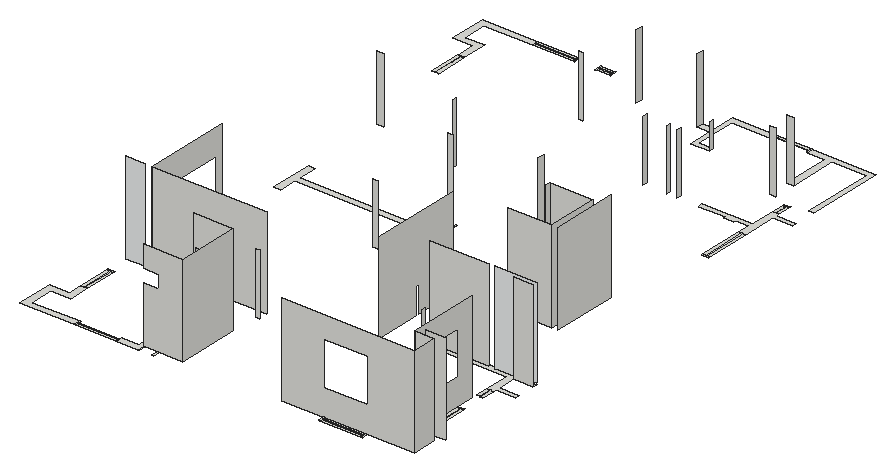
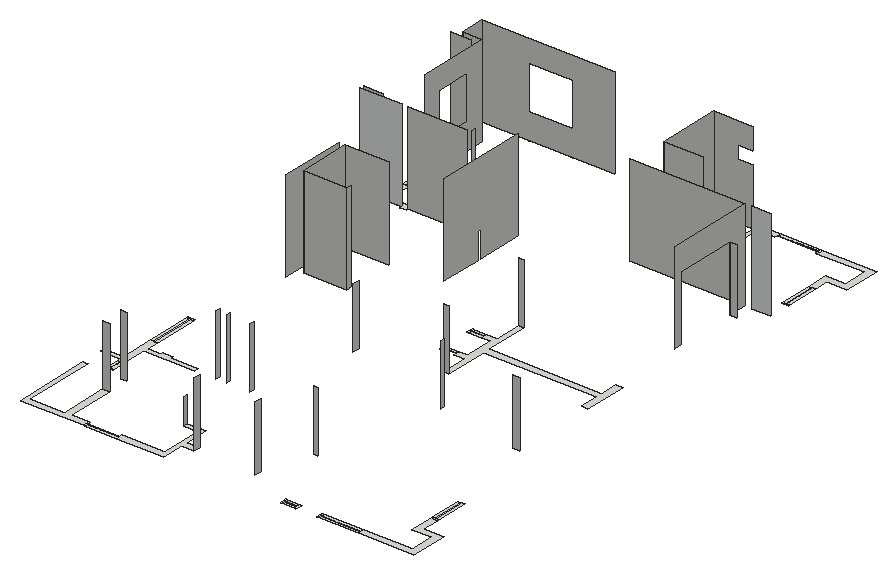
# SketchUp Ruby script. Lengths in inches.
U = 1.inch
M = Sketchup.active_model
def pt(a) = Geom::Point3d.new(a.map { |v| v * U })
def face(e, loops, mat)
  f = e.add_face(loops[0].map { |a| pt(a) })
  loops[1..].each { |l| e.add_face(l.map { |a| pt(a) }).erase! }
  f.material = f.back_material = mat if mat
  f
end
# faces: each face lists its corners as indices into pts; further lists are holes
def faces(e, pts, list, mat = nil) = list.each { |f| face(e, (f[0].is_a?(Array) ? f : [f]).map { |l| l.map { |i| pts[i] } }, mat) }
# xy, xz, yz: faces in a plane at the given z, y or x. An outline is a flat list of corners, or four numbers for a rectangle; further outlines are holes
def ring(l) = l.size == 4 ? [[l[0], l[1]], [l[2], l[1]], [l[2], l[3]], [l[0], l[3]]] : l.each_slice(2).to_a
def flat(e, list, mat, &to3) = list.each { |f| face(e, (f[0].is_a?(Array) ? f : [f]).map { |l| ring(l).map { |u, v| to3.(u, v) } }, mat) }
def xy(e, z, list, mat = nil) = flat(e, list, mat) { |x, y| [x, y, z] }
def xz(e, y, list, mat = nil) = flat(e, list, mat) { |x, z| [x, y, z] }
def yz(e, x, list, mat = nil) = flat(e, list, mat) { |y, z| [x, y, z] }
def lines(e, pts, list) = list.each { |a, b| e.add_line(pt(pts[a]), pt(pts[b])) }
# prism: a flat outline (further loops are holes) pulled along v
def prism(e, loops, v, mat = nil)
  f = face(e, loops, mat); d = Geom::Vector3d.new(v.map { |x| x * U })
  f.pushpull(f.normal.samedirection?(d) ? d.length : -d.length)
end
def box(e, o, s, mat = nil) = prism(e, [[o, [o[0] + s[0], o[1], o[2]], [o[0] + s[0], o[1] + s[1], o[2]], [o[0], o[1] + s[1], o[2]]]], [0, 0, s[2]], mat)
def at(x, y, z, deg = 0) = Geom::Transformation.translation(pt([x, y, z])) * Geom::Transformation.rotation(ORIGIN, Z_AXIS, deg.degrees)
def axes(o, x, y, z) = Geom::Transformation.new([*x, 0, *y, 0, *z, 0, *pt(o).to_a, 1])
def part(name) = M.definitions.add(name)
# library, detail: a bought-in or finely detailed component or shape, given as its bounding box
def library(name, o, s) = part(name).tap { |d| box(d.entities, o, s) }
def detail(e, o, s) = box(e.add_group.entities, o, s)
def put(e, d, t, mat = nil) = e.add_instance(d, t).tap { |i| i.material = mat if mat }
def group(e, t, mat = nil) = e.add_group.tap { |g| g.transformation = t; g.material = mat if mat }.entities
root = M.entities
M.materials.add("[3P0081_White-City]").color = [235, 238, 238]
xy(root,132,[[144,357.97,144,408.97,171,408.97,171,428.87,180,428.87,180,399.97,153,399.97,153,366.97,218,366.97,218,357.97],[218,357.97,220,366.97],[220,357.97,276,361.97],[276,357.97,276,366.97,300,366.97,300,459.97,309,459.97,309,453.97,306,453.97,306,357.97],[306,357.97,308,366.97],
  [325.5,357.97,327.5,366.97],[554.5,357.97,556.5,366.97],[556.5,357.97,612.5,361.97],[612.5,357.97,614.5,366.97],[220,361.97,276,362.97],
  [556.5,361.97,612.5,362.97],[556.5,362.97,612.5,366.97],[652.5,426.87,661.5,428.87],[171,428.87,175,472.87],[175,428.87,176,472.87],
  [176,428.87,180,472.87],[652.5,428.87,656.5,472.87],[656.5,428.87,657.5,472.87],[657.5,428.87,661.5,472.87],[171,472.87,180,474.87],
  [652.5,472.87,661.5,474.87],[539,498.97,539,504.97,541.5,504.97,541.5,564.97,622.5,564.97,622.5,567.97,631.5,567.97,631.5,564.97,688.5,564.97,688.5,558.97,661.5,558.97,661.5,535,688.5,535,688.5,529,661.5,529,661.5,524.53,652.5,524.53,652.5,558.97,547.5,558.97,547.5,504.97,553.5,504.97,553.5,498.97],[652.5,507.03,656.5,524.53],[656.5,507.03,657.5,524.53],[657.5,507.03,661.5,524.53],
  [363,690.97,363,750.97,207,750.97,207,726.97,198,726.97,198,785.97,207,785.97,207,759.97,363,759.97,363,819.97,369,819.97,369,783.97,384.75,783.97,384.75,774.97,372,774.97,372,735.97,384.75,735.97,384.75,726.97,369,726.97,369,690.97],[384.75,726.97,402.25,730.97],[402.25,726.97,404.25,735.97],[384.75,730.97,402.25,731.97],[384.75,731.97,402.25,735.97],
  [384.75,774.97,402.25,778.97],[402.25,774.97,404.25,783.97],[384.75,778.97,402.25,779.97],[649.5,897.97,658.5,899.97],[649.5,899.97,653.5,961.97],
  [653.5,899.97,654.5,961.97],[654.5,899.97,658.5,961.97],[649.5,961.97,649.5,978.97,631.5,978.97,631.5,975.97,617.5,975.97,617.5,978.97,580.5,978.97,580.5,984.97,649.5,984.97,649.5,1019.47,658.5,1019.47,658.5,1015,685.5,1015,685.5,1009,658.5,1009,658.5,961.97],[649.5,1019.47,653.5,1036.97],[653.5,1019.47,654.5,1036.97],
  [654.5,1019.47,658.5,1036.97],[171,1031.97,175,1075.97],[175,1031.97,176,1075.97],[176,1031.97,180,1075.97],[649.5,1036.97,658.5,1038.97],
  [679.5,1044.97,679.5,1143.97,631.5,1143.97,631.5,1077.97,622.5,1077.97,622.5,1143.97,598.5,1143.97,598.5,1152.97,685.5,1152.97,685.5,1044.97],[171,1075.97,180,1077.97],[171,1077.97,171,1101.97,144,1101.97,144,1152.97,220,1152.97,220,1143.97,153,1143.97,153,1110.97,180,1110.97,180,1077.97],[487.5,1080.97,487.5,1113.97,470.25,1113.97,470.25,1122.97,487.5,1122.97,487.5,1152.97,552.5,1152.97,552.5,1143.97,493.5,1143.97,493.5,1086.97,513.5,1086.97,513.5,1080.97],[220,1143.97,276,1147.97],
  [276,1143.97,278,1152.97],[306,1143.97,308,1152.97],[308,1143.97,325.5,1147.97],[325.5,1143.97,327.5,1152.97],[596.5,1143.97,598.5,1152.97],
  [220,1147.97,276,1148.97],[308,1147.97,325.5,1148.97],[552.5,1147.97,596.5,1148.97],[220,1148.97,276,1152.97],[308,1148.97,325.5,1152.97],
  [552.5,1148.97,596.5,1152.97]])
xz(root,366.97,[[306,132,306,210,327.5,210,327.5,228,306,228,306,258,360,258,360,132],[[496.5,132,679.5,258],[554.5,168,614.5,228]]])
xz(root,399.97,[[652.5,132,679.5,258]])
xz(root,408.97,[[661.5,132,688.5,258]])
xz(root,453.97,[[306,132,309,132,309,216,333,216,333,132,360,132,360,258,306,258]])
xz(root,492.97,[[360,132,366,216]])
xz(root,504.97,[[207,132,366,258]])
xz(root,504.97,[[171,132,198,258]],"[3P0081_White-City]")
xz(root,530.97,[[198,132,207,222]])
xz(root,558.97,[[661.5,132,688.5,258]])
xz(root,564.97,[[541.5,132,622.5,258]])
xz(root,564.97,[[631.5,132,631.5,258,688.5,258,688.5,134,682.5,134,682.5,132]],"[3P0081_White-City]")
xz(root,672.97,[[562.5,132,622.5,258]])
xz(root,690.97,[[363,132,369,216]])
xz(root,744.97,[[562.5,132,622.5,258]])
xz(root,819.97,[[363,132,369,216]])
xz(root,903.97,[[198,132,207,222]])
xz(root,1047.47,[[360,132,366,216]])
xz(root,1047.97,[[622.5,132,631.5,216]])
xz(root,1077.97,[[622.5,132,631.5,216]])
yz(root,207,[[504.97,132,530.97,132,530.97,222,614.97,222,614.97,132,624.97,132,624.97,258,504.97,258]])
yz(root,309,[[453.97,132,459.97,216]])
yz(root,321,[[879.97,132,885.97,216]])
yz(root,333,[[453.97,132,459.97,216]])
yz(root,360,[[366.97,132,453.97,258]])
yz(root,386.25,[[1113.97,132,1122.97,222]])
yz(root,470.25,[[1113.97,132,1122.97,222]])
yz(root,472.5,[[837.97,132,846.97,216]])
yz(root,493.5,[[537.97,132,600.97,132,600.97,168,606.97,168,606.97,132,663.97,132,663.97,258,537.97,258]])
yz(root,504,[[978.97,132,984.97,216]])
yz(root,513.5,[[1080.97,132,1086.97,168]])
yz(root,536,[[978.97,132,984.97,216]])
yz(root,550.5,[[978.97,132,984.97,216]])
yz(root,562.5,[[741.97,132,744.97,132,744.97,258,738.97,258,738.97,134,741.97,134]])
yz(root,583.5,[[498.97,132,504.97,216]])
yz(root,622.5,[[672.97,132,744.97,258]])
yz(root,631.5,[[672.97,132,763.97,258]])
yz(root,652.5,[[[399.97,132,498.97,258],[426.87,168,474.87,228]]])
yz(root,679.5,[[366.97,132,399.97,258]])
